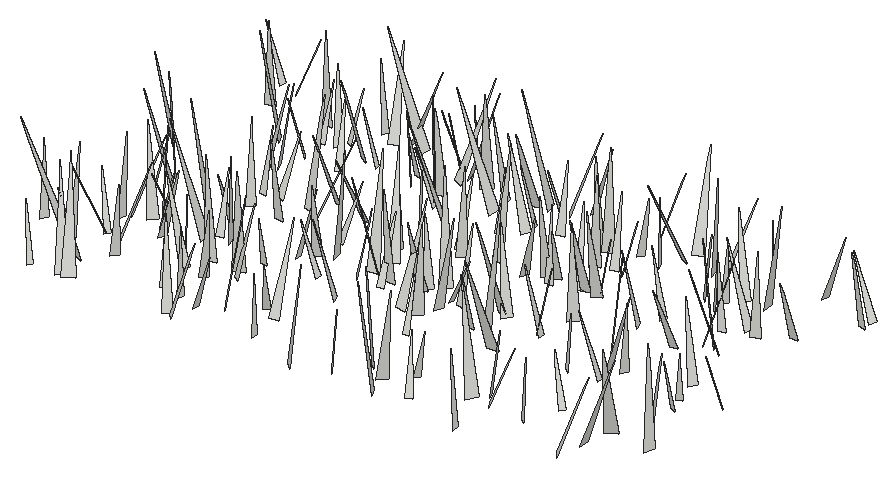
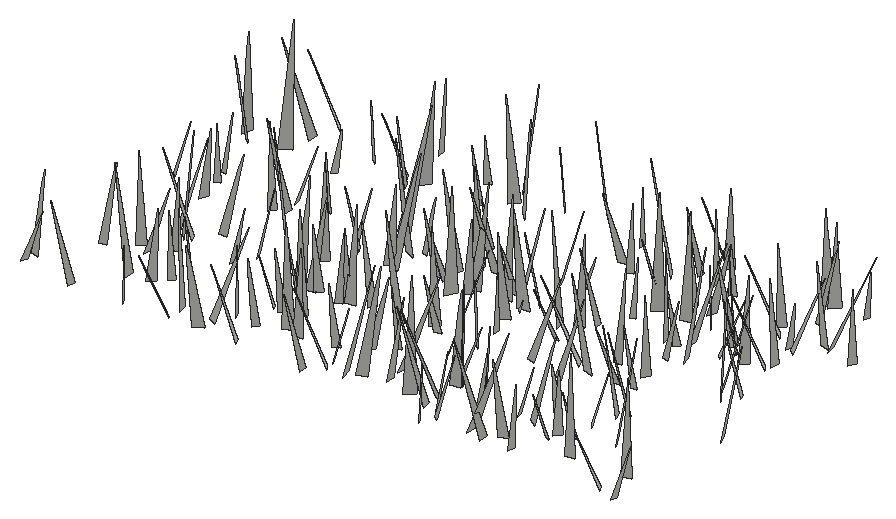
# SketchUp Ruby script. Lengths in inches.
U = 1.inch
M = Sketchup.active_model
def pt(a) = Geom::Point3d.new(a.map { |v| v * U })
def face(e, loops, mat)
  f = e.add_face(loops[0].map { |a| pt(a) })
  loops[1..].each { |l| e.add_face(l.map { |a| pt(a) }).erase! }
  f.material = f.back_material = mat if mat
  f
end
# faces: each face lists its corners as indices into pts; further lists are holes
def faces(e, pts, list, mat = nil) = list.each { |f| face(e, (f[0].is_a?(Array) ? f : [f]).map { |l| l.map { |i| pts[i] } }, mat) }
# xy, xz, yz: faces in a plane at the given z, y or x. An outline is a flat list of corners, or four numbers for a rectangle; further outlines are holes
def ring(l) = l.size == 4 ? [[l[0], l[1]], [l[2], l[1]], [l[2], l[3]], [l[0], l[3]]] : l.each_slice(2).to_a
def flat(e, list, mat, &to3) = list.each { |f| face(e, (f[0].is_a?(Array) ? f : [f]).map { |l| ring(l).map { |u, v| to3.(u, v) } }, mat) }
def xy(e, z, list, mat = nil) = flat(e, list, mat) { |x, y| [x, y, z] }
def xz(e, y, list, mat = nil) = flat(e, list, mat) { |x, z| [x, y, z] }
def yz(e, x, list, mat = nil) = flat(e, list, mat) { |y, z| [x, y, z] }
def lines(e, pts, list) = list.each { |a, b| e.add_line(pt(pts[a]), pt(pts[b])) }
# prism: a flat outline (further loops are holes) pulled along v
def prism(e, loops, v, mat = nil)
  f = face(e, loops, mat); d = Geom::Vector3d.new(v.map { |x| x * U })
  f.pushpull(f.normal.samedirection?(d) ? d.length : -d.length)
end
def box(e, o, s, mat = nil) = prism(e, [[o, [o[0] + s[0], o[1], o[2]], [o[0] + s[0], o[1] + s[1], o[2]], [o[0], o[1] + s[1], o[2]]]], [0, 0, s[2]], mat)
def at(x, y, z, deg = 0) = Geom::Transformation.translation(pt([x, y, z])) * Geom::Transformation.rotation(ORIGIN, Z_AXIS, deg.degrees)
def axes(o, x, y, z) = Geom::Transformation.new([*x, 0, *y, 0, *z, 0, *pt(o).to_a, 1])
def part(name) = M.definitions.add(name)
# library, detail: a bought-in or finely detailed component or shape, given as its bounding box
def library(name, o, s) = part(name).tap { |d| box(d.entities, o, s) }
def detail(e, o, s) = box(e.add_group.entities, o, s)
def put(e, d, t, mat = nil) = e.add_instance(d, t).tap { |i| i.material = mat if mat }
def group(e, t, mat = nil) = e.add_group.tap { |g| g.transformation = t; g.material = mat if mat }.entities
root = M.entities
c1 = part("fur_instance\#9")
p = [[0.8125,0,1.79],[0.67,-0.02,1.48],[0,-0.11,0],[0,0.11,0]]
faces(c1.entities,p,[[0,1,2,3]])
put(root,c1,axes([526.03,108.74,-21.66],[-5.05567,-0.39861,1.84756],[-0.46846,5.37567,-0.1221],[1.83109,0.27472,5.06989]))
put(root,c1,axes([500.86,108.43,-21.66],[4.54729,4.68314,2.12923],[4.88324,-4.82336,0.17985],[-1.61844,-1.39522,6.52513]))
put(root,c1,axes([461.32,108.42,-21.66],[-3.55756,1.9012,0.49829],[1.88183,3.59228,-0.2708],[0.56709,0.00632,4.02461]))
put(root,c1,axes([512.83,109.45,-21.66],[-6.35073,-3.49942,2.22612],[-3.7296,6.59945,-0.26567],[1.81428,1.31702,7.24617]))
put(root,c1,axes([482.47,108.76,-21.66],[3.7464,3.46532,0.67043],[3.46985,-3.79505,0.22613],[-0.64655,-0.28736,5.09832]))
put(root,c1,axes([481.64,109.23,-21.66],[-3.36286,5.21282,1.50099],[5.38655,3.41774,0.19865],[0.64152,-1.37145,6.20023]))
put(root,c1,axes([465.86,108.84,-21.66],[-5.00326,5.02156,1.24961],[5.08502,5.09325,-0.10752],[0.95924,-0.80806,7.08781]))
put(root,c1,axes([466.94,108.77,-21.66],[-4.81371,6.17541,1.55135],[6.27572,4.93015,-0.15223],[1.07597,-1.1279,7.82843]))
put(root,c1,axes([505.83,110.44,-21.66],[3.13173,2.6382,1.54856],[2.8558,-3.31576,-0.12654],[-1.0966,-1.10068,4.0929]))
put(root,c1,axes([493.28,111.34,-21.66],[-3.94466,-0.14605,1.57067],[-0.23954,4.23653,-0.20765],[1.55915,0.28136,3.94189]))
put(root,c1,axes([464.99,113.09,-21.66],[-2.33347,-4.94017,0.88075],[-4.99474,2.38012,0.11709],[0.48332,0.74554,5.4623]))
put(root,c1,axes([511.69,112.67,-21.66],[5.17414,-4.36417,1.70527],[-4.54977,-5.28673,0.27499],[-1.1196,1.31532,6.76329]))
put(root,c1,axes([517,111.08,-21.66],[-1.66344,3.87519,0.54462],[3.91265,1.65754,0.1564],[0.06977,-0.56232,4.21422]))
put(root,c1,axes([483.39,112.48,-21.66],[4.21997,-0.6182,0.41958],[-0.60999,-4.24047,-0.11271],[-0.43142,-0.05127,4.26352]))
put(root,c1,axes([539.4,111.39,-21.66],[4.3993,3.63087,0.47155],[3.65139,-4.40515,-0.14642],[-0.27004,-0.41338,5.70225]))
put(root,c1,axes([480.38,113.27,-21.66],[4.66089,-0.94094,1.87831],[-0.93791,-5.02216,-0.1885],[-1.87983,0.17273,4.75118]))
put(root,c1,axes([508.77,114.47,-21.66],[-4.32305,-4.69404,2.5219],[-5.10648,4.57733,-0.23372],[1.52244,2.02405,6.37716]))
put(root,c1,axes([477.3,114.02,-21.66],[-1.55614,3.71904,0.91385],[3.82438,1.56093,0.15988],[0.20123,-0.90564,4.0283]))
put(root,c1,axes([486.06,114.77,-21.66],[6.38411,4.40631,2.11358],[4.61615,-6.57865,-0.22824],[-1.60436,-1.39477,7.75373]))
put(root,c1,axes([514.53,115.77,-21.66],[2.97768,-2.23657,0.59018],[-2.29034,-2.98547,0.24174],[-0.32391,0.5494,3.71623]))
put(root,c1,axes([531.14,115.26,-21.66],[2.46567,3.17158,1.58955],[3.37143,-2.69731,0.15219],[-1.10413,-1.15357,4.01439]))
put(root,c1,axes([540.26,115.43,-21.66],[6.68807,0.43229,0.66728],[0.41432,-6.71942,0.20043],[-0.67859,0.15798,6.69903]))
put(root,c1,axes([467.89,116.36,-21.66],[3.7544,-3.60472,1.46029],[-3.77286,-3.86843,0.15082],[-0.94444,1.12393,5.20257]))
put(root,c1,axes([490.26,117.45,-21.66],[1.67975,-3.93598,0.16611],[-3.93538,-1.66827,0.26597],[0.17974,0.25696,4.27115]))
put(root,c1,axes([522.85,115.84,-21.66],[-6.40886,3.74132,2.19702],[3.96061,6.64492,0.23769],[1.77143,-1.32114,7.41717]))
put(root,c1,axes([525.56,115.78,-21.66],[3.83341,2.26597,0.28943],[2.28132,-3.82668,-0.25597],[-0.11822,-0.36786,4.44568]))
put(root,c1,axes([459.98,116.95,-21.66],[-7.66892,-1.90839,0.15613],[-1.91216,7.66661,-0.21311],[0.09999,0.24454,7.89993]))
put(root,c1,axes([541.15,119.54,-21.66],[4.3126,-6.65441,0.44802],[-6.65528,-4.32849,-0.22777],[-0.435,0.25174,7.9264]))
put(root,c1,axes([460.99,116.96,-21.66],[1.59622,5.71911,2.00108],[6.0184,-1.73595,0.16062],[-0.70101,-1.88115,5.93551]))
put(root,c1,axes([524.24,117.64,-21.66],[4.12014,1.91723,1.34742],[2.03951,-4.27599,-0.15214],[-1.154,-0.71202,4.54182]))
put(root,c1,axes([479.39,118.95,-21.66],[3.84963,-3.94903,0.87916],[-4.01863,-3.87266,0.20133],[-0.4673,0.77142,5.51126]))
put(root,c1,axes([492.52,116,-21.66],[-0.48607,6.36101,0.33267],[6.36907,0.48063,0.1158],[-0.09028,-0.34048,6.37851]))
put(root,c1,axes([455.69,118.21,-21.66],[-4.75498,1.70819,1.94206],[1.76287,5.11453,-0.18234],[1.89256,-0.47231,5.04921]))
put(root,c1,axes([463.16,120.43,-21.66],[-3.18461,-4.17271,0.10236],[-4.17132,3.18622,0.10881],[0.1486,0.01532,5.24799]))
put(root,c1,axes([547.39,119.05,-21.66],[6.19428,-1.57461,3.33029],[-1.87234,-6.95675,0.19327],[-3.17247,1.03131,6.38836]))
put(root,c1,axes([466.87,118.07,-21.66],[4.58247,4.01128,0.43645],[4.00699,-4.60163,0.22113],[-0.47421,-0.12046,6.08609]))
put(root,c1,axes([476.4375,119.09,-21.66],[-5.80582,1.67481,0.45332],[1.66732,5.82342,-0.1609],[0.48013,0.02943,6.04042]))
put(root,c1,axes([463.92,119.87,-21.66],[-3.60805,2.068,0.36238],[2.05277,3.62596,-0.25393],[0.44056,0.04128,4.15092]))
put(root,c1,axes([533.08,120.24,-21.66],[-2.90723,2.3787,0.42473],[2.40963,2.90345,0.23285],[0.1797,-0.4498,3.74913]))
put(root,c1,axes([546.18,120.66,-21.66],[3.88828,4.27161,1.82836],[4.44707,-4.1121,0.14976],[-1.3465,-1.2459,5.77433]))
put(root,c1,axes([481.9375,122.43,-21.66],[3.60415,-6.43604,2.10161],[-6.7075,-3.71823,0.11619],[-0.92131,1.89247,7.37557]))
put(root,c1,axes([474.4375,121.8,-21.66],[2.87799,2.64757,1.74089],[2.94858,-3.09885,-0.16173],[-1.16026,-1.30792,3.90721]))
put(root,c1,axes([477.77,122.375,-21.66],[1.68119,-6.78383,2.85706],[-7.30642,-1.89388,-0.19753],[-0.89411,2.72073,6.98625]))
put(root,c1,axes([482.83,120.95,-21.66],[2.64907,4.14771,0.84835],[4.17625,-2.72433,0.27885],[-0.69438,-0.56151,4.91358]))
put(root,c1,axes([469.53,123.48,-21.66],[5.0608,-1.8582,0.79428],[-1.91101,-5.09708,0.2516],[-0.65714,0.51221,5.38529]))
put(root,c1,axes([517.55,126.52,-21.66],[0.59961,-8.00132,0.48644],[-8.01433,-0.60861,-0.13198],[-0.1682,0.47514,8.02267]))
put(root,c1,axes([507.09,122.93,-21.66],[-0.85461,3.70026,0.75554],[3.7566,0.91253,-0.21994],[0.38824,-0.68446,3.79129]))
put(root,c1,axes([495.14,124.44,-21.66],[-4.90258,-2.23132,0.87524],[-2.28191,4.95484,-0.15015],[0.73329,0.50088,5.38438]))
put(root,c1,axes([462.8,124.09,-21.66],[5.47635,-0.94494,2.24683],[-1.1073,-5.8869,0.22307],[-2.17142,0.61884,5.55279]))
put(root,c1,axes([483.2,125.73,-21.66],[0.28978,-3.77503,0.68612],[-3.83038,-0.24462,0.27184],[0.22308,0.70349,3.77636]))
put(root,c1,axes([468.47,124.68,-21.66],[-4.89725,-3.9807,3.26033],[-4.56553,5.43754,-0.21877],[2.37312,2.24631,6.30723]))
put(root,c1,axes([468.35,124.48,-21.66],[2.84043,2.51238,0.82611],[2.52394,-2.93724,0.2547],[-0.79009,-0.35083,3.78354]))
put(root,c1,axes([469.16,126.7,-21.66],[-2.85386,-2.94003,0.13695],[-2.93623,2.85714,0.14971],[0.2028,-0.00613,4.09462]))
put(root,c1,axes([473.71,126.33,-21.66],[-7.9003,-1.05971,0.99848],[-1.05239,7.96314,0.1246],[1.0062,0.00826,7.97008]))
put(root,c1,axes([465.95,126.08,-21.66],[-4.07853,4.6775,2.02917],[4.97181,4.22458,0.25488],[1.13033,-1.70436,6.20068]))
put(root,c1,axes([463.3,125.36,-21.66],[4.56753,3.50086,0.36537],[3.49009,-4.58212,0.27435],[-0.45689,-0.00383,5.74831]))
put(root,c1,axes([490.24,127.28,-21.66],[-3.8674,0.14725,0.40736],[0.1724,3.88071,0.23399],[0.39736,-0.25058,3.86312]))
put(root,c1,axes([505.23,127.54,-21.66],[-4.12278,4.06528,3.37823],[4.64279,4.83304,-0.14992],[2.52655,-2.24755,5.78803]))
put(root,c1,axes([476.7,127.56,-21.66],[5.38301,1.51294,2.42188],[1.75431,-5.82988,-0.25732],[-2.2532,-0.92457,5.58566]))
put(root,c1,axes([543.37,128.57,-21.66],[-0.97443,-3.66118,0.75209],[-3.71136,1.03977,0.25308],[0.44234,0.6588,3.78017]))
put(root,c1,axes([527.48,128.1,-21.66],[-2.04031,-2.94511,1.87891],[-3.25881,2.38849,0.20512],[1.25863,1.41005,3.57693]))
put(root,c1,axes([512.32,129.02,-21.66],[-1.30736,-3.53096,1.01989],[-3.67333,1.2908,-0.2398],[0.12042,1.04076,3.75757]))
put(root,c1,axes([532.06,128.74,-21.66],[-4.50006,-1.01814,0.39176],[-1.03948,4.50642,-0.22865],[0.331,0.31016,4.60813]))
put(root,c1,axes([474.9,127.68,-21.66],[-1.60634,4.05647,0.77587],[4.09581,1.67158,-0.25963],[0.53033,-0.623,4.35521]))
put(root,c1,axes([471.78,129.73,-21.66],[-7.67624,-2.38765,2.18106],[-2.53698,7.93,-0.24775],[2.0054,0.89261,8.03519]))
put(root,c1,axes([502.64,127.42,-21.66],[0.72086,7.11073,0.81641],[7.15729,-0.71063,-0.13028],[0.04812,-0.82534,7.14599]))
put(root,c1,axes([485.32,129.64,-21.66],[5.08569,0.11573,0.95874],[0.07501,-5.17107,0.22632],[-0.96278,0.20845,5.08197]))
put(root,c1,axes([502,132.36,-21.66],[2.77965,-6.05851,0.20454],[-6.05263,-2.78627,-0.276],[-0.3362,0.0706,6.66001]))
put(root,c1,axes([486.8125,131.42,-21.66],[3.24454,-4.71501,1.03025],[-4.7617,-3.32972,-0.24278],[-0.78672,0.70811,5.71834]))
put(root,c1,axes([506.35,130.21,-21.66],[6.38697,-1.69717,1.73981],[-1.81592,-6.58358,0.24416],[-1.61547,0.69051,6.6041]))
put(root,c1,axes([473.87,131.15,-21.66],[-0.63245,-3.70623,0.66325],[-3.76509,0.62047,-0.12308],[-0.01169,0.67448,3.75779]))
put(root,c1,axes([542.48,130.83,-21.66],[1.6475,-3.20979,0.84583],[-3.31321,-1.64761,0.20101],[-0.20196,0.8456,3.6023]))
put(root,c1,axes([493.76,130.26,-21.66],[4.05853,2.67005,1.15678],[2.78357,-4.14094,-0.20805],[-0.84796,-0.81387,4.85361]))
put(root,c1,axes([497.67,131.63,-21.66],[0.14601,-6.62439,2.10053],[-6.94709,-0.08453,0.21629],[0.18059,2.1039,6.62247]))
put(root,c1,axes([531.47,131.14,-21.66],[5.98361,0.11352,0.76596],[0.13466,-6.02993,-0.15823],[-0.76252,-0.17402,5.9826]))
put(root,c1,axes([513.71,130.26,-21.66],[3.41828,7.22194,2.57308],[7.56489,-3.63472,0.1519],[-1.24484,-2.25703,7.98861]))
put(root,c1,axes([533.1875,132.01,-21.66],[4.53528,-3.04969,1.17101],[-3.07507,-4.66168,-0.23091],[-1.10265,0.45689,5.46041]))
put(root,c1,axes([495.05,132.64,-21.66],[-4.80805,-4.95386,1.3489],[-5.02147,4.92244,0.17909],[1.0701,0.84054,6.90116]))
put(root,c1,axes([497.5,130.03,-21.66],[-0.4926,4.67354,0.05511],[4.67276,0.49124,0.10792],[-0.10156,-0.0661,4.69819]))
put(root,c1,axes([513.0625,134,-21.66],[-2.01035,-7.12989,1.00319],[-7.18316,2.0575,0.22838],[0.49393,0.90254,7.40437]))
put(root,c1,axes([547.67,132.6,-21.66],[-2.17535,-3.01047,0.60266],[-3.06621,2.16789,-0.23847],[0.15643,0.62897,3.70651]))
put(root,c1,axes([463.9,132.75,-21.66],[-6.35383,-3.10693,1.06991],[-3.1587,6.41685,-0.12448],[0.9057,0.58302,7.07168]))
put(root,c1,axes([488.82,132.6,-21.66],[7.15031,1.42356,2.57616],[1.59453,-7.56218,-0.24693],[-2.47399,-0.75958,7.28646]))
put(root,c1,axes([506.3,132.55,-21.66],[3.59656,-0.31618,0.04156],[-0.31764,-3.59357,0.14939],[-0.02828,0.15246,3.60734]))
put(root,c1,axes([519.87,132.79,-21.66],[-4.57594,-0.69447,0.70937],[-0.73517,4.61906,-0.2203],[0.6671,0.32667,4.62309]))
put(root,c1,axes([461.07,132.58,-21.66],[3.50621,1.98379,0.78234],[2.0421,-3.55715,-0.13217],[-0.61424,-0.50223,4.02634]))
put(root,c1,axes([502.26,133.3125,-21.66],[2.60909,-3.89298,2.22887],[-4.24925,-2.97119,-0.21539],[-1.4377,1.71676,4.68148]))
put(root,c1,axes([507.89,132.31,-21.66],[0.83118,5.18677,1.07004],[5.28228,-0.88982,0.21009],[-0.38088,-1.02179,5.24874]))
put(root,c1,axes([519,133.09,-21.66],[-3.23487,-1.73884,2.61208],[-2.22596,3.91581,-0.14997],[2.2117,1.39779,3.66954]))
put(root,c1,axes([494.65,132.3,-21.66],[-1.18605,7.62635,1.82441],[7.84154,1.15487,0.27022],[0.00582,-1.84431,7.7133]))
put(root,c1,axes([513.9,133.71,-21.66],[-4.47005,3.93119,1.60818],[4.11701,4.5843,0.23722],[1.04438,-1.24571,5.94805]))
put(root,c1,axes([462.84,134.38,-21.66],[-5.77727,-4.35757,2.82703],[-4.73437,6.15702,-0.18467],[2.13687,1.8601,7.23403]))
put(root,c1,axes([477.77,135.41,-21.66],[-0.39451,-5.89979,1.57703],[-6.09619,0.47415,0.24879],[0.36204,1.55494,5.90773]))
put(root,c1,axes([528.8,134.95,-21.66],[5.52113,3.74347,2.2115],[4.00437,-5.77059,-0.2291],[-1.6939,-1.44011,6.66663]))
put(root,c1,axes([541.49,134.71,-21.66],[-4.9618,2.41645,1.1014],[2.44275,5.06865,-0.11597],[1.04177,-0.37582,5.51772]))
put(root,c1,axes([503.73,134.72,-21.66],[5.91163,-3.56463,4.13587],[-4.286,-6.80601,0.26026],[-3.38262,2.39395,6.89828]))
put(root,c1,axes([473.07,135.875,-21.66],[3.99343,-3.31881,2.86458],[-3.84361,-4.5142,0.12826],[-2.10878,1.94301,5.19091]))
put(root,c1,axes([487.09,135.4375,-21.66],[1.39427,3.92432,0.17719],[3.92808,-1.39069,-0.10895],[0.04345,-0.20342,4.16322]))
put(root,c1,axes([495.04,135.53,-21.66],[-2.95766,6.66869,1.17233],[6.76114,2.97762,0.11972],[0.36439,-1.12067,7.29416]))
put(root,c1,axes([520.61,138,-21.66],[4.6761,-4.10232,2.76945],[-4.45315,-5.14998,-0.1096],[-2.16064,1.73593,6.21956]))
put(root,c1,axes([533.99,140.49,-21.66],[0.26999,-5.16111,0.17986],[-5.16087,-0.27616,-0.17741],[-0.18667,0.17024,5.16512]))
put(root,c1,axes([493.77,138.58,-21.66],[-4.03311,-0.04964,1.55556],[-0.10181,4.31995,-0.1261],[1.55302,0.15428,4.03144]))
put(root,c1,axes([486.14,141.46,-21.66],[-1.09873,-5.30096,0.04279],[-5.29764,1.09638,-0.20521],[-0.19227,0.08352,5.40974]))
put(root,c1,axes([481.14,138.38,-21.66],[5.4364,3.24485,0.19999],[3.25087,-5.4295,-0.27539],[-0.03035,-0.33899,6.32516]))
put(root,c1,axes([472.36,139,-21.66],[0.52075,4.40411,1.27547],[4.58416,-0.47433,-0.2338],[0.09203,-1.29345,4.42863]))
put(root,c1,axes([474.73,139.33,-21.66],[0.96438,4.41888,0.40988],[4.43511,-0.94495,-0.24768],[0.15571,-0.45288,4.5161]))
put(root,c1,axes([479.1,139.42,-21.66],[1.99412,7.08431,1.8343],[7.27705,-2.12036,0.27805],[-0.77249,-1.68678,7.35436]))
put(root,c1,axes([538.9,142.65,-21.66],[-4.24041,-4.62675,0.86788],[-4.65391,4.29598,0.16351],[0.70788,0.52807,6.27385]))
put(root,c1,axes([480.99,142.6875,-21.66],[-2.16973,-4.86696,0.63571],[-4.9077,2.16207,-0.19771],[0.07681,0.6613,5.32503]))
put(root,c1,axes([456.41,142.1,-21.66],[-5.55068,-3.03255,1.58004],[-3.06213,5.7489,0.27653],[1.52193,0.50669,6.31901]))
put(root,c1,axes([500.48,141.88,-21.66],[3.75494,-4.9741,2.2471],[-5.32599,-3.93562,0.18806],[-1.1937,1.91308,6.22943]))
put(root,c1,axes([527.41,141.84,-21.66],[-4.67685,-1.64881,1.07356],[-1.71505,4.77313,-0.14071],[0.96421,0.49258,4.95698]))
put(root,c1,axes([509.15,143.03,-21.66],[4.77577,-2.2799,0.31782],[-2.26651,-4.78515,-0.26858],[-0.40236,-0.10607,5.28524]))
put(root,c1,axes([519.17,144.26,-21.66],[2.40943,-6.40182,1.38295],[-6.51779,-2.4885,-0.16399],[-0.64358,1.23501,6.83826]))
put(root,c1,axes([493.33,142.78,-21.66],[2.79577,3.11606,1.7882],[3.42019,-3.00212,-0.11591],[-1.09992,-1.41467,4.18482]))
put(root,c1,axes([517.26,144.54,-21.66],[0.8568,-5.86099,0.80486],[-5.91149,-0.87995,-0.11477],[-0.231,0.77949,5.92218]))
put(root,c1,axes([511.58,144.0625,-21.66],[1.49133,-6.04191,1.54576],[-6.23212,-1.50337,0.13646],[-0.23383,1.53405,6.22175]))
put(root,c1,axes([512.8125,144.81,-21.66],[2.32528,-3.90872,0.2043],[-3.90658,-2.33236,-0.15975],[-0.24182,0.09371,4.54527]))
put(root,c1,axes([537.51,143.61,-21.66],[-5.07554,-4.81191,2.50581],[-5.17107,5.32884,-0.24106],[1.64121,1.90882,6.98981]))
put(root,c1,axes([512.68,143.2,-21.66],[-0.37436,4.96388,1.61425],[5.21969,0.34743,0.14211],[-0.02763,-1.62026,4.97594]))
put(root,c1,axes([536.22,143.35,-21.66],[5.52496,2.9641,0.73245],[3.00682,-5.54515,-0.24054],[-0.53047,-0.55942,6.26523]))
put(root,c1,axes([499.2,142.96,-21.66],[-0.62067,4.74172,0.56344],[4.77083,0.63973,-0.12835],[0.20124,-0.5417,4.78044]))
put(root,c1,axes([504.53,143.68,-21.66],[0.76042,7.54721,2.45249],[7.93568,-0.724,-0.23253],[-0.00259,-2.46349,7.58186]))
put(root,c1,axes([495.14,145.74,-21.66],[-6.81995,-3.62088,0.84533],[-3.65528,6.85252,-0.13797],[0.68141,0.51893,7.72033]))
put(root,c1,axes([468.87,144.3,-21.66],[3.65147,4.43575,1.22236],[4.5601,-3.69672,-0.20725],[-0.61278,-1.07778,5.74161]))
put(root,c1,axes([516.36,144.11,-21.66],[-2.91757,4.706,0.99504],[4.75363,2.9987,-0.24403],[0.73452,-0.71423,5.53165]))
put(root,c1,axes([518.86,145.26,-21.66],[3.30079,2.00098,0.99665],[2.11543,-3.37049,-0.23912],[-0.72261,-0.72685,3.85253]))
put(root,c1,axes([528.85,144.94,-21.66],[-4.50468,1.1443,0.55643],[1.12699,4.53841,-0.20945],[0.5907,0.0676,4.64302]))
put(root,c1,axes([469.8,145.43,-21.66],[5.42096,2.25752,1.64956],[2.38588,-5.61122,-0.16143],[-1.45775,-0.7887,5.87002]))
put(root,c1,axes([536.05,147.04,-21.66],[-1.45922,4.42701,2.15741],[4.90506,1.50733,0.22462],[0.43952,-2.12407,4.65589]))
put(root,c1,axes([540.0625,148.39,-21.66],[2.8988,-5.16102,2.16058],[-5.5292,-3.01461,0.21733],[-0.85564,1.9958,5.91539]))
put(root,c1,axes([470.66,149.2,-21.66],[-3.26871,-2.2439,0.63682],[-2.29753,3.28654,-0.21245],[0.40248,0.53729,3.95909]))
put(root,c1,axes([490.34,149.42,-21.66],[-3.97846,-0.22397,0.26493],[-0.21326,3.98441,0.16592],[0.27363,-0.15114,3.9813]))
put(root,c1,axes([543.85,150.94,-21.66],[0.47232,-5.02453,0.37853],[-5.03579,-0.45765,0.20889],[0.17316,0.39615,5.04235]))
put(root,c1,axes([514.4,149.86,-21.66],[4.01557,-5.25956,2.05629],[-5.53772,-4.16187,0.169],[-1.10676,1.74125,6.61508]))
put(root,c1,axes([500.37,148.91,-21.66],[0.04059,4.23783,1.33242],[4.44047,0.00019,-0.13586],[0.12965,-1.33303,4.23585]))
put(root,c1,axes([538.44,149.25,-21.66],[-5.80532,1.01557,0.17125],[1.00882,5.80466,-0.22508],[0.20737,0.19232,5.88918]))
put(root,c1,axes([465.71,150.6,-21.66],[-6.16765,-3.82155,1.90605],[-3.98751,6.35208,-0.16723],[1.52874,1.15063,7.2537]))
put(root,c1,axes([532.24,150.36,-21.66],[-2.65775,-2.55388,1.91088],[-2.80676,3.05414,0.17806],[1.51521,1.17784,3.68161]))
put(root,c1,axes([476.0625,149,-21.66],[-2.52047,3.62206,0.22803],[3.61381,2.53037,-0.24846],[0.33426,-0.04477,4.40572]))
put(root,c1,axes([489.03,150.83,-21.66],[4.97701,4.02381,2.97396],[4.34378,-5.5566,0.24873],[-2.48337,-1.65505,6.3953]))
put(root,c1,axes([518.21,150.36,-21.66],[2.97809,2.23148,0.68885],[2.24903,-3.04112,0.12836],[-0.62921,-0.30835,3.71915]))
put(root,c1,axes([489.35,151.93,-21.66],[1.40139,-5.88916,2.09043],[-6.21682,-1.53152,-0.14692],[-0.635,1.99706,6.05182]))
put(root,c1,axes([516.77,150.59,-21.66],[-2.07994,4.49979,1.08625],[4.57933,2.1742,-0.23818],[0.67657,-0.88257,4.95151]))
put(root,c1,axes([484.82,151.73,-21.66],[-3.86454,-2.68359,1.87384],[-2.96857,4.09497,-0.25773],[1.3786,1.29506,4.69786]))
put(root,c1,axes([502.83,151.22,-21.66],[-5.78073,2.46703,0.60773],[2.49572,5.79658,0.20851],[0.47643,-0.43109,6.28168]))
put(root,c1,axes([476.64,153.01,-21.66],[-2.84226,-5.05917,1.08036],[-5.16298,2.85167,-0.22901],[0.32566,1.05526,5.79838]))
put(root,c1,axes([529.49,151.88,-21.66],[3.10895,3.01642,1.49943],[3.22004,-3.26039,-0.11754],[-0.98914,-1.13301,4.33019]))
put(root,c1,axes([531.97,152.69,-21.66],[2.86459,-3.18276,1.27512],[-3.34476,-2.95943,0.1272],[-0.754,1.03614,4.28015]))
put(root,c1,axes([479.02,152.6,-21.66],[-3.86057,-0.50737,0.50019],[-0.53854,3.88252,-0.21837],[0.46646,0.28336,3.88764]))
put(root,c1,axes([496.76,152.7,-21.66],[-8.06825,0.70999,0.37952],[0.71569,8.07597,0.10667],[0.36866,-0.13964,8.09873]))
put(root,c1,axes([484.07,153.95,-21.66],[-0.05824,-3.81958,0.55077],[-3.85535,0.08183,0.15984],[0.16986,0.54776,3.81668]))
put(root,c1,axes([502.81,153.0625,-21.66],[-3.79015,-1.11399,0.60809],[-1.15598,3.82064,-0.20588],[0.52388,0.37109,3.9451]))
put(root,c1,axes([513.49,153.54,-21.66],[-2.45983,6.23998,3.07468],[6.83629,2.77173,-0.15592],[1.28687,-2.79677,6.7055]))
put(root,c1,axes([506.4,153.25,-21.66],[-1.7521,4.37342,1.24469],[4.49457,1.86786,-0.23622],[0.6891,-1.06311,4.7054]))
put(root,c1,axes([511.42,154.29,-21.66],[-0.9402,5.50023,2.63792],[6.09336,0.97222,0.14463],[0.28664,-2.62629,5.57814]))
put(root,c1,axes([470.32,152.92,-21.66],[0.12612,4.07155,0.3622],[4.08216,-0.1442,0.19951],[-0.2114,-0.35539,4.06861]))
put(root,c1,axes([499.63,156.82,-21.66],[2.0561,-6.44135,0.2848],[-6.4395,-2.06652,-0.24899],[-0.32395,0.19535,6.75697]))
put(root,c1,axes([472.42,153.5,-21.66],[-4.08375,3.22336,1.0157],[3.24667,4.18417,-0.22495],[0.93853,-0.4488,5.19774]))
put(root,c1,axes([520.35,154.82,-21.66],[4.15283,1.56186,1.94961],[1.7605,-4.5132,-0.13443],[-1.7723,-0.82343,4.43479]))
put(root,c1,axes([536.68,155.05,-21.66],[7.17764,0.6661,2.04171],[0.73913,-7.45363,-0.1667],[-2.01642,-0.36113,7.20655]))
put(root,c1,axes([517.06,155.3125,-21.66],[3.70956,-2.15387,1.10856],[-2.28011,-3.78925,0.26761],[-0.81802,0.79458,4.28116]))
put(root,c1,axes([496.37,155.54,-21.66],[-5.73495,-0.11109,1.68244],[-0.04447,5.97258,0.24275],[1.68552,-0.22038,5.73089]))
put(root,c1,axes([533.68,154.54,-21.66],[-4.18107,4.06515,1.12452],[4.17237,4.21812,0.26475],[0.61747,-0.97641,5.82552]))
put(root,c1,axes([521.83,157.65,-21.66],[-3.10911,-5.59083,0.18925],[-5.58666,3.11434,0.22319],[0.28707,0.05678,6.39328]))
put(root,c1,axes([492.43,156.6875,-21.66],[4.53182,-5.76132,1.66498],[-5.89155,-4.66684,-0.11276],[-1.12014,1.237,7.32923]))
put(root,c1,axes([504.39,156.33,-21.66],[-3.02688,-2.08558,0.64094],[-2.07151,3.09116,0.27563],[0.68504,0.13224,3.66547]))
put(root,c1,axes([459.58,156.42,-21.66],[2.04038,-5.82637,1.87095],[-6.1057,-2.07021,0.21174],[-0.4092,1.83789,6.16967]))
put(root,c1,axes([472.86,154.93,-21.66],[1.48501,3.27806,0.44782],[3.28348,-1.52047,0.24164],[-0.40618,-0.30651,3.59062]))
put(root,c1,axes([468,156.81,-21.66],[0.12589,-6.48138,2.39431],[-6.90548,-0.03647,0.26437],[0.23531,2.39734,6.47721]))
put(root,c1,axes([501.4,157.74,-21.66],[-7.78363,-1.77881,1.5879],[-1.77027,7.9428,0.22014],[1.59741,0.13482,7.98126]))
put(root,c1,axes([548.46,158.27,-21.66],[-1.20745,-5.31811,1.49773],[-5.50418,1.29079,0.14593],[0.47907,1.42653,5.45151]))
put(root,c1,axes([526.46,157.6,-21.66],[-5.78196,-1.74059,3.08913],[-1.82129,6.52793,0.26926],[3.04225,0.59997,6.03227]))
put(root,c1,axes([487.04,158.375,-21.66],[2.58883,2.26123,2.35644],[2.87323,-3.00647,-0.27159],[-1.55259,-1.79333,3.42658]))
put(root,c1,axes([488.87,155.63,-21.66],[3.08355,6.47581,0.56476],[6.50039,-3.07095,-0.27862],[0.00972,-0.62967,7.16706]))
put(root,c1,axes([489.17,157.61,-21.66],[6.39922,1.66084,0.77373],[1.68967,-6.43637,-0.15871],[-0.70856,-0.34898,6.60932]))
put(root,c1,axes([486.41,159.37,-21.66],[-2.51428,-3.3921,0.48717],[-3.39486,2.54791,0.21985],[0.4675,0.25907,4.21659]))
put(root,c1,axes([481.19,158.86,-21.66],[-8.2127,0.65784,0.53458],[0.66874,8.22786,0.14871],[0.52088,-0.19122,8.23766]))
put(root,c1,axes([504.21,157.84,-21.66],[4.71146,3.59222,0.48874],[3.58656,-4.73541,0.23065],[-0.52868,-0.11206,5.92019]))
put(root,c1,axes([478.84,159.61,-21.66],[6.32916,0.13104,0.27334],[0.13733,-6.3333,-0.14369],[-0.27023,-0.14945,6.32889]))
put(root,c1,axes([477.09,158.07,-21.66],[-2.49742,5.95651,1.04282],[6.02179,2.55284,-0.16018],[0.55273,-0.89868,6.45689]))
put(root,c1,axes([474.625,159.54,-21.66],[-4.53937,1.16522,1.40638],[1.15678,4.75002,-0.2018],[1.41333,-0.14527,4.6822]))
put(root,c1,axes([516.41,159.71,-21.66],[4.75078,2.28793,0.55209],[2.32197,-4.75936,-0.25743],[-0.38451,-0.47246,5.26671]))
put(root,c1,axes([506.1,160.03,-21.66],[4.91416,0.05831,0.74386],[0.02898,-4.96646,0.19783],[-0.74558,0.19125,4.91052]))
put(root,c1,axes([548.78,159.89,-21.66],[-4.27711,1.68369,0.0136],[1.68167,4.26988,0.26227],[-0.08344,-0.24902,4.58909]))
put(root,c1,axes([533.05,160.57,-21.66],[3.08289,1.97486,1.70839],[2.08981,-3.45082,0.21788],[-1.56569,-0.71742,3.6547]))
put(root,c1,axes([540.625,161.13,-21.66],[5.32067,-0.59583,0.38531],[-0.58759,-5.33383,-0.13414],[-0.39777,-0.09079,5.35224]))
put(root,c1,axes([487.4,161.2,-21.66],[2.96101,1.91002,1.7712],[2.18546,-3.28075,-0.11568],[-1.41742,-1.06838,3.5217]))
put(root,c1,axes([526.92,159.79,-21.66],[2.95968,3.81178,0.17357],[3.80838,-2.96454,0.16477],[-0.23661,-0.0359,4.82309]))
put(root,c1,axes([457.63,161.37,-21.66],[-4.13289,0.76106,0.51137],[0.79822,4.14817,0.27763],[0.45116,-0.36746,4.1932]))
put(root,c1,axes([460.37,160.43,-21.66],[3.48298,2.03603,0.22687],[2.02285,-3.48877,0.25421],[-0.32396,0.10555,4.02641]))
put(root,c1,axes([522.31,159.71,-21.66],[-2.78795,6.31949,0.96814],[6.36227,2.84625,-0.25738],[0.62828,-0.78026,6.90234]))
